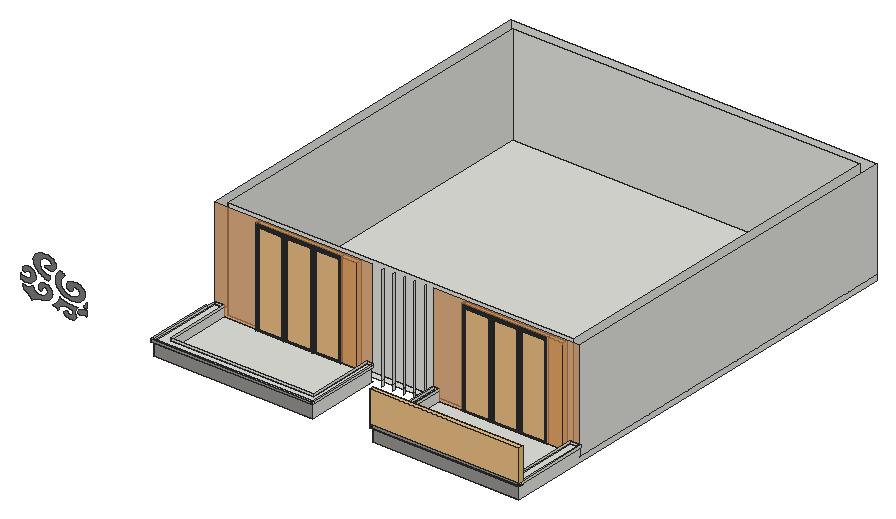
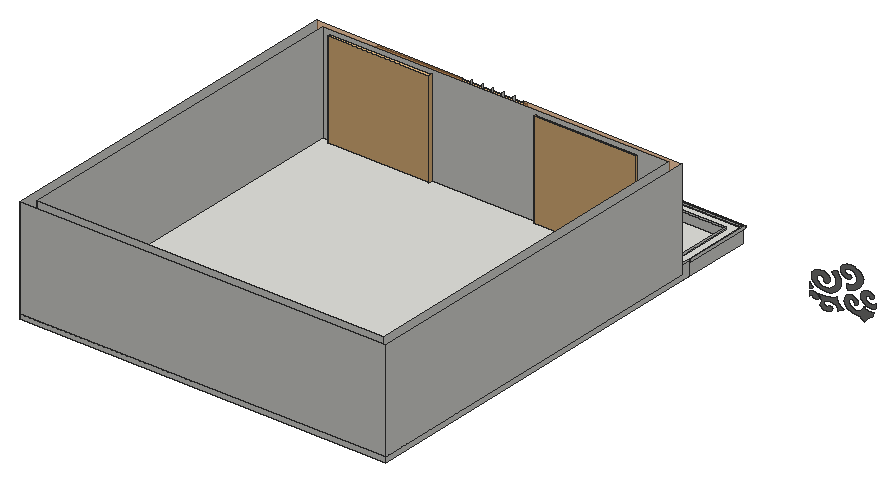
# SketchUp Ruby script. Lengths in inches.
U = 1.inch
M = Sketchup.active_model
def pt(a) = Geom::Point3d.new(a.map { |v| v * U })
def face(e, loops, mat)
  f = e.add_face(loops[0].map { |a| pt(a) })
  loops[1..].each { |l| e.add_face(l.map { |a| pt(a) }).erase! }
  f.material = f.back_material = mat if mat
  f
end
# faces: each face lists its corners as indices into pts; further lists are holes
def faces(e, pts, list, mat = nil) = list.each { |f| face(e, (f[0].is_a?(Array) ? f : [f]).map { |l| l.map { |i| pts[i] } }, mat) }
# xy, xz, yz: faces in a plane at the given z, y or x. An outline is a flat list of corners, or four numbers for a rectangle; further outlines are holes
def ring(l) = l.size == 4 ? [[l[0], l[1]], [l[2], l[1]], [l[2], l[3]], [l[0], l[3]]] : l.each_slice(2).to_a
def flat(e, list, mat, &to3) = list.each { |f| face(e, (f[0].is_a?(Array) ? f : [f]).map { |l| ring(l).map { |u, v| to3.(u, v) } }, mat) }
def xy(e, z, list, mat = nil) = flat(e, list, mat) { |x, y| [x, y, z] }
def xz(e, y, list, mat = nil) = flat(e, list, mat) { |x, z| [x, y, z] }
def yz(e, x, list, mat = nil) = flat(e, list, mat) { |y, z| [x, y, z] }
def lines(e, pts, list) = list.each { |a, b| e.add_line(pt(pts[a]), pt(pts[b])) }
# prism: a flat outline (further loops are holes) pulled along v
def prism(e, loops, v, mat = nil)
  f = face(e, loops, mat); d = Geom::Vector3d.new(v.map { |x| x * U })
  f.pushpull(f.normal.samedirection?(d) ? d.length : -d.length)
end
def box(e, o, s, mat = nil) = prism(e, [[o, [o[0] + s[0], o[1], o[2]], [o[0] + s[0], o[1] + s[1], o[2]], [o[0], o[1] + s[1], o[2]]]], [0, 0, s[2]], mat)
def at(x, y, z, deg = 0) = Geom::Transformation.translation(pt([x, y, z])) * Geom::Transformation.rotation(ORIGIN, Z_AXIS, deg.degrees)
def axes(o, x, y, z) = Geom::Transformation.new([*x, 0, *y, 0, *z, 0, *pt(o).to_a, 1])
def part(name) = M.definitions.add(name)
# library, detail: a bought-in or finely detailed component or shape, given as its bounding box
def library(name, o, s) = part(name).tap { |d| box(d.entities, o, s) }
def detail(e, o, s) = box(e.add_group.entities, o, s)
def put(e, d, t, mat = nil) = e.add_instance(d, t).tap { |i| i.material = mat if mat }
def group(e, t, mat = nil) = e.add_group.tap { |g| g.transformation = t; g.material = mat if mat }.entities
root = M.entities
M.materials.add("Wine2").color = [0, 0, 0]
M.materials["Wine2"].alpha = 0
M.materials.add("[0043_SaddleBrown]4").color = [124, 123, 122]
M.materials.add("[0130_Gainsboro]").color = [39, 45, 50]
M.materials.add("[Granite Light Gray]").color = [149, 148, 144]
M.materials.add("[Wood Floor Light]").color = [204, 176, 127]
M.materials.add("[Wood Floor]").color = [224, 152, 88]
M.materials["[Wood Floor]"].alpha = 0.68
c1 = part("Framed glazing panel")
xy(c1.entities,0,[[0,-0.98,43.07,0],[0,0,43.07,1.4]],"[0130_Gainsboro]")
xy(c1.entities,0.3,[[0.3,-1.43,42.77,-0.98]],"[0130_Gainsboro]")
xy(c1.entities,2.95,[[2.95,-1.43,40.12,-0.63],[2.95,-0.63,40.12,0],[2.95,0,40.12,0.64],[2.95,0.64,40.12,1.4]],"[0130_Gainsboro]")
xy(c1.entities,3.54,[[3.54,-0.63,39.53,0],[3.54,0,39.53,0.64]],"[0130_Gainsboro]")
xy(c1.entities,111.8125,[[3.54,-0.63,39.53,0],[3.54,0,39.53,0.64]],"[0130_Gainsboro]")
xy(c1.entities,112.4,[[2.95,-1.43,40.12,-0.63],[2.95,-0.63,40.12,0],[2.95,0,40.12,0.64],[2.95,0.64,40.12,1.4]],"[0130_Gainsboro]")
xy(c1.entities,115.05,[[0.3,-1.43,42.77,-0.98]],"[0130_Gainsboro]")
xy(c1.entities,115.35,[[0,-0.98,43.07,0],[0,0,43.07,1.4]],"[0130_Gainsboro]")
xz(c1.entities,-1.43,[[[0.3,0.3,42.77,115.05],[2.95,2.95,40.12,112.4]]],"[0130_Gainsboro]")
xz(c1.entities,-0.98,[[[0,0,43.07,115.35],[0.3,0.3,42.77,115.05]]],"[0130_Gainsboro]")
xz(c1.entities,-0.63,[[[2.95,2.95,40.12,112.4],[3.54,3.54,39.53,111.8125]]],"[0130_Gainsboro]")
xz(c1.entities,0,[[3.54,3.54,39.53,111.8125]],"Wine2")
xz(c1.entities,0,[[[0,0,43.07,115.35],[2.95,2.95,40.12,112.4]],[[2.95,2.95,40.12,112.4],[3.54,3.54,39.53,111.8125]]],"[0130_Gainsboro]")
xz(c1.entities,0.64,[[[2.95,2.95,40.12,112.4],[3.54,3.54,39.53,111.8125]]],"[0130_Gainsboro]")
xz(c1.entities,1.4,[[[0,0,43.07,115.35],[2.95,2.95,40.12,112.4]]],"[0130_Gainsboro]")
yz(c1.entities,0,[[-0.98,0,0,115.35],[0,0,1.4,115.35]],"[0130_Gainsboro]")
yz(c1.entities,0.3,[[-1.43,0.3,-0.98,115.05]],"[0130_Gainsboro]")
yz(c1.entities,2.95,[[-1.43,2.95,-0.63,112.4],[-0.63,2.95,0,112.4],[0,2.95,0.64,112.4],[0.64,2.95,1.4,112.4]],"[0130_Gainsboro]")
yz(c1.entities,3.54,[[-0.63,3.54,0,111.8125],[0,3.54,0.64,111.8125]],"[0130_Gainsboro]")
yz(c1.entities,39.53,[[-0.63,3.54,0,111.8125],[0,3.54,0.64,111.8125]],"[0130_Gainsboro]")
yz(c1.entities,40.12,[[-1.43,2.95,-0.63,112.4],[-0.63,2.95,0,112.4],[0,2.95,0.64,112.4],[0.64,2.95,1.4,112.4]],"[0130_Gainsboro]")
yz(c1.entities,42.77,[[-1.43,0.3,-0.98,115.05]],"[0130_Gainsboro]")
yz(c1.entities,43.07,[[-0.98,0,0,115.35],[0,0,1.4,115.35]],"[0130_Gainsboro]")
c2 = part("Glazing assembly")
put(c2.entities,c1,axes([90.57,1.43,0],[1.05148,0,0],[0,1,0],[0,0,1]))
put(c2.entities,c1,axes([0,1.43,0],[1.05148,0,0],[0,1,0],[0,0,1]))
put(c2.entities,c1,axes([45.29,1.43,0],[1.05148,0,0],[0,1,0],[0,0,1]))
c3 = library("Curtains",[0,0,0],[121.73,8.19,117.22])
c4 = library("Glass Railing",[0,0,0],[139.5,4.76,42])
xy(root,388.875,[[1852.64,651.03,1953.89,657.03],[2100.38,651.03,2201.63,657.03]])
xy(root,394.4375,[[1802.38,559.875,1993.07,570.83],[2065.52,559.875,2240.81,570.83],[1813.71,657.03,2229.49,1085.17]])
xy(root,394.4375,[[1802.38,570.83,1813.71,651.03],[1813.71,570.83,1993.07,651.03],[2065.52,570.83,2229.49,651.03],[2229.49,570.83,2240.81,651.03]],"[Wood Floor Light]")
xy(root,400.4375,[[1813.71,570.83,1985.21,570.83,1985.21,651.03,1953.89,651.03,1953.89,657.03,1852.64,657.03,1852.64,651.03,1813.71,651.03],[2071.59,570.83,2229.49,570.83,2229.49,651.03,2201.63,651.03,2201.63,657.03,2100.38,657.03,2100.38,651.03,2071.59,651.03],[1802.38,651.03,1802.38,1096.5,2240.81,1096.5,2240.81,651.03,2201.63,651.03,2201.63,657.03,2229.49,657.03,2229.49,1085.17,1813.71,1085.17,1813.71,657.03,1852.64,657.03,1852.64,651.03],[1813.71,657.03,2229.49,1085.17]])
xy(root,410.625,[[1800.63,557.9375,1993.07,559.875],[1993.07,557.9375,1995.01,559.875],[2063.58,557.9375,2065.52,559.875],[2065.52,557.9375,2240.81,559.875],[2240.81,557.9375,2242.75,559.875],
  [1800.45,559.875,1802.38,640.11],[1802.38,559.875,1802.38,651.03,1813.71,651.03,1813.71,570.83,1985.21,570.83,1985.21,651.03,1993.07,651.03,1993.07,559.875],[1993.07,559.875,1995.01,647.91],[2063.58,559.875,2065.52,651.03],[2065.52,559.875,2065.52,651.03,2071.59,651.03,2071.59,570.83,2229.49,570.83,2229.49,651.03,2240.81,651.03,2240.81,559.875],
  [2240.81,559.875,2242.75,651.03]])
xz(root,557.9375,[[2240.81,410.625,2242.75,413.5]])
xz(root,557.9375,[[1800.63,410.625,1993.07,413.5],[1993.07,410.625,1995.01,413.5],[2063.58,410.625,2065.52,413.5],[2065.52,410.625,2240.81,413.5]],"[Granite Light Gray]")
xz(root,559.875,[[1800.45,410.625,1800.63,413.5],[1800.63,410.625,1802.38,413.5],[1802.38,410.625,1993.07,413.5],[1993.07,410.625,1995.01,413.5],[2063.58,410.625,2065.52,413.5],
  [2065.52,410.625,2240.81,413.5],[2240.81,410.625,2242.75,413.5]])
xz(root,559.875,[[1802.38,394.4375,1993.07,410.625],[2065.52,394.4375,2240.81,410.625]],"[Granite Light Gray]")
xz(root,570.83,[[1813.71,400.4375,1985.21,410.625],[2071.59,400.4375,2229.49,410.625],[1813.71,410.625,1985.21,413.5],[2071.59,410.625,2229.49,413.5]])
xz(root,589.17,[[1678.15,378.34,1679.8125,378.37,1681.43,378.64,1682.9375,379.15,1684.27,379.86,1685.37,380.76,1686.19,381.8,1685.625,382.74,1685.18,383.71,1684.86,384.71,1684.65,385.72,1684.58,386.75,1684.63,387.77,1684.81,388.79,1685.11,389.79,1685.53,390.76,1686.07,391.71,1686.72,392.62,1687.49,393.48,1685.61,393.37,1683.72,393.33,1681.84,393.38,1679.96,393.5,1678.1,393.71,1676.25,393.99,1674.43,394.35,1672.65,394.79,1670.9,395.3,1669.2,395.88,1667.55,396.54,1665.95,397.26,1665.83,396.19,1665.6,395.13,1665.26,394.09,1664.82,393.07,1664.26,392.07,1663.61,391.11,1662.86,390.1875,1662.02,389.31,1661.08,388.47,1660.0625,387.69,1658.97,386.97,1657.8,386.31,1658.42,386.1,1659.03,385.89,1659.64,385.67,1660.23,385.44,1660.83,385.2,1661.99,384.7,1662.56,384.44,1663.13,384.16,1663.6875,383.88,1664.23,383.59,1664.77,383.3,1664.88,384.7,1665.41,386.05,1666.33,387.29,1667.6,388.35,1669.16,389.19,1670.94,389.77,1672.85,390.05,1674.8,390.03,1676.69,389.7,1678.44,389.08,1679.96,388.2,1681.18,387.11,1681.22,386.77,1681.24,386.43,1681.25,386.09,1681.24,385.75,1681.22,385.41,1681.18,385.07,1681.13,384.73,1681.07,384.39,1680.99,384.06,1680.9,383.72,1680.79,383.39,1680.67,383.06,1680.08,382.875,1679.45,382.76,1678.8,382.72,1678.16,382.75,1677.52,382.85,1676.92,383.03,1676.37,383.27,1675.88,383.58,1675.46,383.93,1675.12,384.33,1674.88,384.76,1674.73,385.22,1674.33,385.09,1673.9375,384.95,1673.56,384.79,1673.19,384.61,1672.84,384.41,1672.51,384.2,1672.2,383.98,1671.91,383.74,1671.64,383.48,1671.39,383.22,1671.17,382.95,1670.97,382.66,1671.55,381.54,1672.44,380.53,1673.6,379.68,1674.98,379.01,1676.52,378.55],[1632.59,382.25,1633.2,383.03,1633.91,383.77,1634.73,384.44,1635.64,385.06,1636.625,385.6,1637.6875,386.07,1638.81,386.46,1639.98,386.77,1641.19,386.98,1642.42,387.11,1643.67,387.15,1644.91,387.09,1647.33,387.5,1649.61,388.2,1651.69,389.18,1653.5,390.4,1654.99,391.84,1656.1,393.4375,1656.82,395.15,1657.1,396.93,1656.96,398.71,1656.38,400.46,1655.39,402.1,1654.02,403.59,1652.9,404.41,1651.55,405.05,1650.06,405.47,1648.47,405.65,1646.86,405.59,1645.3125,405.29,1643.89,404.75,1642.64,404.02,1641.65,403.11,1640.93,402.07,1640.54,400.95,1640.48,399.79,1640.54,399.43,1640.65,399.08,1640.82,398.73,1641.03,398.4,1641.28,398.09,1641.58,397.8,1641.92,397.53,1642.3,397.29,1642.71,397.08,1643.14,396.9,1643.6,396.75,1644.08,396.64,1644.16,397.15,1644.29,397.65,1644.45,398.15,1644.65,398.64,1644.9,399.13,1645.18,399.6,1645.5,400.06,1645.85,400.5,1646.24,400.93,1646.67,401.34,1647.125,401.74,1647.61,402.11,1648.55,401.77,1649.4,401.34,1650.15,400.81,1650.77,400.2,1651.26,399.54,1651.61,398.83,1651.79,398.08,1651.82,397.33,1651.68,396.58,1651.39,395.86,1650.94,395.18,1650.35,394.55,1649.52,393.61,1648.45,392.8,1647.19,392.14,1645.79,391.66,1644.29,391.38,1642.74,391.3,1641.2,391.43,1639.72,391.76,1638.35,392.28,1637.13,392.98,1636.12,393.82,1635.33,394.79,1635.12,395.05,1634.92,395.3125,1634.72,395.58,1634.54,395.85,1634.22,396.41,1634.08,396.69,1633.84,397.27,1633.74,397.5625,1633.65,397.86,1633.58,398.15,1632.88,397.49,1632.08,396.89,1631.19,396.375,1630.21,395.94,1629.16,395.6,1628.0625,395.35,1626.93,395.2,1625.78,395.16,1624.63,395.22,1623.5,395.38,1622.41,395.64,1621.375,396,1621.59,395.6875,1621.78,395.37,1621.95,395.04,1622.09,394.71,1622.2,394.375,1622.29,394.03,1622.35,393.6875,1622.38,393.34,1622.38,392.99,1622.36,392.65,1622.31,392.3,1622.23,391.96,1623.37,391.33,1624.47,390.67,1625.52,389.96,1626.53,389.22,1627.48,388.45,1628.38,387.64,1629.23,386.81,1630.02,385.95,1630.76,385.06,1631.43,384.14,1632.04,383.2],[1690.69,386.82,1691.23,386.85,1691.7,386.92,1692.15,387.02,1692.59,387.15,1693.01,387.31,1693.41,387.49,1693.78,387.7,1694.13,387.93,1694.45,388.18,1694.74,388.45,1694.99,388.74,1695.2,389.05,1695.38,389.36,1695.73,389.23,1696.0625,389.09,1696.4,388.93,1696.72,388.77,1697.34,388.43,1697.64,388.24,1697.93,388.05,1698.21,387.85,1698.48,387.65,1698.74,387.4375,1698.99,387.22,1698.99,393,1698.02,393.38,1696.97,393.65,1695.88,393.8,1694.77,393.8125,1693.67,393.7,1692.61,393.47,1691.62,393.11,1690.71,392.65,1689.92,392.09,1689.26,391.45,1688.76,390.73,1688.41,389.97,1688.16,389.63,1688,389.25,1687.95,388.86,1688,388.47,1688.15,388.09,1688.4,387.74,1688.74,387.4375,1689.16,387.18,1689.63,386.99,1690.15,386.87],[1698.61,396.46,1698.99,396.47,1698.99,402.56,1698.71,402.125,1698.42,401.6875,1698.11,401.26,1697.8,400.83,1697.47,400.41,1697.13,399.99,1696.78,399.58,1696.41,399.18,1696.04,398.77,1695.65,398.38,1695.25,397.99,1694.85,397.61,1695.12,397.42,1695.42,397.24,1695.73,397.08,1696.05,396.9375,1696.39,396.8125,1696.74,396.71,1697.1,396.62,1697.47,396.55,1697.85,396.5,1698.23,396.47],[1680.49,398.78,1682.69,398.88,1684.85,399.21,1686.93,399.74,1688.89,400.47,1690.7,401.39,1692.31,402.47,1693.71,403.7,1694.86,405.0625,1695.74,406.52,1696.34,408.05,1696.64,409.625,1696.64,410.99,1696.36,412.35,1695.8,413.65,1694.99,414.89,1693.93,416.03,1692.66,417.04,1691.19,417.91,1689.57,418.61,1687.82,419.14,1685.98,419.47,1684.09,419.61,1682.2,419.54,1680.72,419.33,1679.32,418.9375,1678.02,418.39,1676.87,417.7,1675.89,416.875,1675.11,415.95,1674.54,414.95,1674.22,413.89,1674.14,412.81,1674.3,411.73,1674.71,410.68,1675.35,409.7,1675.87,409.31,1676.48,409,1677.17,408.79,1677.91,408.68,1678.66,408.6875,1679.4,408.8,1680.09,409.03,1680.69,409.35,1681.2,409.75,1681.57,410.22,1681.81,410.73,1681.7,411.09,1681.64,411.45,1681.63,411.81,1681.6875,412.17,1681.8,412.52,1681.96,412.87,1682.18,413.19,1682.44,413.5,1682.75,413.79,1683.11,414.04,1683.5,414.27,1683.92,414.46,1684.93,414.36,1685.91,414.15,1686.83,413.83,1687.67,413.41,1688.41,412.9,1689.04,412.32,1689.53,411.68,1689.88,410.98,1690.08,410.26,1690.125,409.53,1690.01,408.8,1689.74,408.08,1689,406.9,1687.99,405.82,1686.74,404.88,1685.29,404.1,1683.6875,403.5,1681.97,403.11,1680.18,402.93,1678.37,402.96,1676.6,403.22,1674.91,403.68,1673.35,404.34,1671.97,405.17,1670.52,406.36,1669.3,407.66,1668.32,409.08,1667.62,410.57,1667.1875,412.12,1667.04,413.7,1667.1875,415.27,1667.62,416.82,1668.32,418.3125,1669.3,419.73,1670.52,421.04,1671.97,422.22,1671.61,422.57,1671.22,422.9,1670.82,423.22,1670.39,423.53,1669.95,423.82,1669.49,424.1,1669.01,424.37,1668.51,424.61,1668,424.84,1667.48,425.06,1666.94,425.25,1666.39,425.43,1665.27,424.36,1664.26,423.23,1663.37,422.04,1662.6,420.8125,1661.97,419.55,1661.46,418.25,1661.1,416.93,1660.86,415.6,1660.77,414.25,1660.82,412.91,1661,411.57,1661.32,410.24,1661.85,408.8125,1662.58,407.43,1663.5,406.1,1664.61,404.85,1665.88,403.69,1667.32,402.63,1668.89,401.68,1670.59,400.85,1672.4,400.15,1674.3,399.58,1676.27,399.16,1678.29,398.88],
  [1625.6,399.74,1626.67,399.78,1627.74,399.9,1628.78,400.1,1629.79,400.36,1630.76,400.7,1632.46,401.49,1633.96,402.47,1635.22,403.61,1636.21,404.88,1636.9,406.25,1637.29,407.68,1637.35,409.14,1637.08,410.58,1636.5,411.98,1635.62,413.29,1634.46,414.48,1633.04,415.52,1632.0625,416.12,1630.95,416.58,1629.73,416.875,1628.45,417,1627.17,416.95,1625.92,416.72,1624.76,416.33,1623.72,415.79,1622.83,415.12,1622.14,414.34,1621.67,413.48,1621.43,412.57,1621.34,412.22,1621.34,411.86,1621.45,411.51,1621.64,411.18,1621.92,410.89,1622.27,410.63,1622.68,410.4375,1623.14,410.3,1623.63,410.24,1624.125,410.24,1624.61,410.31,1625.07,410.45,1625.34,410.7,1625.625,410.9375,1625.93,411.17,1626.26,411.38,1626.61,411.58,1626.97,411.76,1627.35,411.92,1627.74,412.07,1628.14,412.2,1628.56,412.31,1628.98,412.4,1629.41,412.47,1629.97,412.12,1630.47,411.73,1630.9,411.29,1631.25,410.82,1631.52,410.32,1631.7,409.8,1631.79,409.27,1631.8,408.74,1631.71,408.2,1631.53,407.69,1631.26,407.1875,1630.91,406.71,1630.1875,406,1629.3,405.39,1628.29,404.89,1627.17,404.53,1625.98,404.3,1624.76,404.23,1623.53,404.3,1622.35,404.53,1621.23,404.89,1620.21,405.39,1619.33,406,1618.6,406.71,1618.6,401.47,1619.48,401.01,1620.41,400.625,1621.39,400.3,1622.41,400.05,1623.45,399.875,1624.52,399.77],[1652.625,409.96,1653.04,410.4,1653.4,410.87,1653.71,411.35,1653.98,411.86,1654.1875,412.37,1654.34,412.89,1654.44,413.42,1654.49,413.96,1654.48,414.49,1654.41,415.03,1654.29,415.56,1654.12,416.08,1652.76,415.96,1651.4,415.98,1650.06,416.14,1648.76,416.43,1647.53,416.85,1646.38,417.38,1645.36,418.02,1644.46,418.76,1643.71,419.58,1643.13,420.47,1642.72,421.4,1642.5,422.37,1642.13,423.29,1641.9,424.22,1641.8125,425.17,1641.87,426.125,1642.06,427.06,1642.39,427.99,1642.86,428.875,1643.45,429.73,1644.17,430.52,1645.01,431.26,1645.94,431.93,1646.98,432.53,1647.93,432.92,1648.98,433.1875,1650.07,433.3,1651.18,433.26,1652.25,433.08,1653.26,432.75,1654.16,432.29,1654.93,431.71,1655.53,431.04,1655.94,430.3,1656.16,429.52,1656.16,428.72,1656.07,428.33,1655.91,427.95,1655.68,427.59,1655.38,427.25,1655.03,426.95,1654.61,426.6875,1654.16,426.46,1653.66,426.29,1653.14,426.16,1652.6,426.09,1652.04,426.07,1651.49,426.11,1650.92,426.125,1650.36,426.05,1649.83,425.88,1649.37,425.63,1649,425.3125,1648.75,424.94,1648.61,424.54,1648.61,424.13,1648.73,423.72,1648.98,423.35,1649.34,423.03,1649.79,422.77,1651.04,422.33,1652.38,422.0625,1653.76,421.97,1655.14,422.0625,1656.48,422.33,1657.73,422.77,1658.84,423.37,1659.79,424.1,1660.53,424.95,1661.06,425.875,1661.33,426.86,1661.36,427.86,1661.41,429.07,1661.24,430.28,1660.83,431.45,1660.21,432.58,1659.375,433.63,1658.35,434.59,1657.15,435.44,1655.8,436.17,1654.33,436.75,1652.76,437.18,1651.12,437.46,1649.44,437.5625,1647.11,437.47,1644.82,437.11,1642.64,436.49,1640.62,435.64,1638.8125,434.58,1637.25,433.32,1635.99,431.9,1635.04,430.36,1634.44,428.73,1634.2,427.05,1634.33,425.37,1634.82,423.72,1635.375,422.12,1636.13,420.56,1637.08,419.06,1638.22,417.63,1639.54,416.28,1641.02,415.02,1642.66,413.87,1644.44,412.83,1646.34,411.91,1648.35,411.12,1650.45,410.47]],"[0043_SaddleBrown]4")
xz(root,640.11,[[1800.45,410.625,1802.38,413.5]])
xz(root,647.91,[[1993.07,410.625,1995.01,413.5]])
xz(root,651.03,[[1802.38,400.4375,1813.71,410.625],[2229.49,400.4375,2240.81,410.625],[1802.38,410.625,1813.71,413.5],[1985.21,410.625,1993.07,413.5],[2063.58,410.625,2065.31,413.5],
  [2065.31,410.625,2065.52,413.5],[2065.52,410.625,2071.59,413.5],[2229.49,410.625,2240.81,413.5],[2240.81,410.625,2242.75,413.5]])
xz(root,651.03,[[1813.71,400.4375,1852.64,400.4375,1852.64,514.875,1953.89,514.875,1953.89,400.4375,1985.21,400.4375,1985.21,413.5,1993.07,413.5,1993.07,520.4375,1802.38,520.4375,1802.38,413.5,1813.71,413.5],[2071.59,400.4375,2100.38,400.4375,2100.38,514.875,2201.63,514.875,2201.63,400.4375,2229.49,400.4375,2229.49,413.5,2240.81,413.5,2240.81,520.4375,2065.52,520.4375,2065.52,413.5,2071.59,413.5]],"[Wood Floor]")
xz(root,657.03,[[1813.71,400.4375,1813.71,520.4375,2229.49,520.4375,2229.49,400.4375,2201.63,400.4375,2201.63,514.875,2100.38,514.875,2100.38,400.4375,1953.89,400.4375,1953.89,514.875,1852.64,514.875,1852.64,400.4375]])
xz(root,1085.17,[[1813.71,400.4375,2229.49,520.4375]])
xz(root,1096.5,[[1802.38,394.4375,2240.81,400.4375],[1802.38,400.4375,2240.81,520.4375]])
yz(root,1800.45,[[559.875,410.625,640.11,413.5]])
yz(root,1800.63,[[557.9375,410.625,559.875,413.5]])
yz(root,1802.38,[[559.875,394.4375,640.11,410.625],[640.11,394.4375,640.11,410.625,651.03,410.625,651.03,400.4375,1096.5,400.4375,1096.5,394.4375],[651.03,400.4375,1096.5,520.4375],[559.875,410.625,640.11,413.5],[640.11,410.625,651.03,413.5]])
yz(root,1813.71,[[570.83,400.4375,651.03,410.625],[657.03,400.4375,1085.17,520.4375],[570.83,410.625,651.03,413.5]])
yz(root,1852.64,[[651.03,400.4375,657.03,514.875]])
yz(root,1953.89,[[651.03,400.4375,657.03,514.875]])
yz(root,1985.21,[[570.83,400.4375,651.03,410.625],[570.83,410.625,651.03,413.5]])
yz(root,1993.07,[[559.875,394.4375,647.91,410.625],[557.9375,410.625,559.875,413.5],[559.875,410.625,647.91,413.5],[647.91,410.625,651.03,413.5]])
yz(root,1995.01,[[557.9375,410.625,559.875,413.5],[559.875,410.625,647.91,413.5]])
yz(root,2006.07,[[647.91,394.4375,651.03,400.4375],[647.91,400.4375,651.03,520.4375]])
yz(root,2018.82,[[648.85,394.4375,651.03,400.4375],[648.85,400.4375,651.03,520.4375]])
yz(root,2030.94,[[648.85,394.4375,651.03,400.4375],[648.85,400.4375,651.03,520.4375]])
yz(root,2043.32,[[648.85,394.4375,651.03,400.4375],[648.85,400.4375,651.03,520.4375]])
yz(root,2056.19,[[648.85,394.4375,651.03,400.4375],[648.85,400.4375,651.03,520.4375]])
yz(root,2063.58,[[557.9375,410.625,559.875,413.5],[559.875,410.625,651.03,413.5]])
yz(root,2065.52,[[559.875,394.4375,651.03,410.625],[557.9375,410.625,559.875,413.5],[559.875,410.625,651.03,413.5]])
yz(root,2071.59,[[570.83,400.4375,651.03,410.625],[570.83,410.625,651.03,413.5]])
yz(root,2100.38,[[651.03,400.4375,657.03,514.875]])
yz(root,2201.63,[[651.03,400.4375,657.03,514.875]])
yz(root,2229.49,[[570.83,400.4375,651.03,410.625],[657.03,400.4375,1085.17,520.4375],[570.83,410.625,651.03,413.5]])
yz(root,2240.81,[[559.875,394.4375,1096.5,394.4375,1096.5,400.4375,651.03,400.4375,651.03,410.625,559.875,410.625],[651.03,400.4375,1096.5,520.4375],[557.9375,410.625,559.875,413.5],[559.875,410.625,651.03,413.5]])
yz(root,2242.75,[[557.9375,410.625,559.875,413.5],[559.875,410.625,651.03,413.5]])
p = [[1681.89,589.17,411.27],[1681.81,589.17,410.73]]
lines(root,p,[[0,1]])
put(root,c2,axes([1852.23,650.7,397.79],[0.75,0,0],[0,0.75,0],[0,0,1.01765]))
put(root,c3,at(1851.45,651.68,397.95))
put(root,c2,axes([2099.73,651.03,397.48],[0.75,0,0],[0,0.75,0],[0,0,1.01765]))
put(root,c4,axes([2063.58,558.12,409.93],[1.28434,0,0],[0,1,0],[0,0,1]),"[Granite Light Gray]")
put(root,c3,at(2098.49,652.22,397.95))
